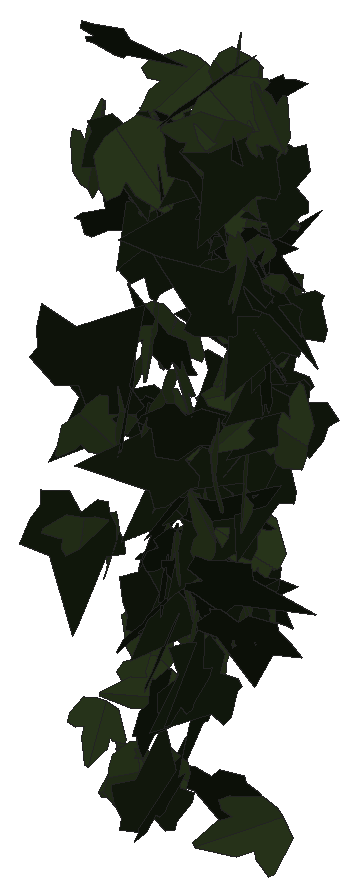
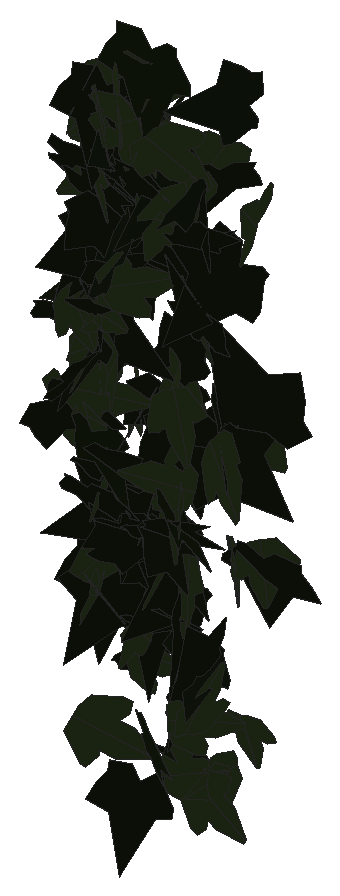
# SketchUp Ruby script. Lengths in inches.
U = 1.inch
M = Sketchup.active_model
def pt(a) = Geom::Point3d.new(a.map { |v| v * U })
def face(e, loops, mat)
  f = e.add_face(loops[0].map { |a| pt(a) })
  loops[1..].each { |l| e.add_face(l.map { |a| pt(a) }).erase! }
  f.material = f.back_material = mat if mat
  f
end
# faces: each face lists its corners as indices into pts; further lists are holes
def faces(e, pts, list, mat = nil) = list.each { |f| face(e, (f[0].is_a?(Array) ? f : [f]).map { |l| l.map { |i| pts[i] } }, mat) }
# xy, xz, yz: faces in a plane at the given z, y or x. An outline is a flat list of corners, or four numbers for a rectangle; further outlines are holes
def ring(l) = l.size == 4 ? [[l[0], l[1]], [l[2], l[1]], [l[2], l[3]], [l[0], l[3]]] : l.each_slice(2).to_a
def flat(e, list, mat, &to3) = list.each { |f| face(e, (f[0].is_a?(Array) ? f : [f]).map { |l| ring(l).map { |u, v| to3.(u, v) } }, mat) }
def xy(e, z, list, mat = nil) = flat(e, list, mat) { |x, y| [x, y, z] }
def xz(e, y, list, mat = nil) = flat(e, list, mat) { |x, z| [x, y, z] }
def yz(e, x, list, mat = nil) = flat(e, list, mat) { |y, z| [x, y, z] }
def lines(e, pts, list) = list.each { |a, b| e.add_line(pt(pts[a]), pt(pts[b])) }
# prism: a flat outline (further loops are holes) pulled along v
def prism(e, loops, v, mat = nil)
  f = face(e, loops, mat); d = Geom::Vector3d.new(v.map { |x| x * U })
  f.pushpull(f.normal.samedirection?(d) ? d.length : -d.length)
end
def box(e, o, s, mat = nil) = prism(e, [[o, [o[0] + s[0], o[1], o[2]], [o[0] + s[0], o[1] + s[1], o[2]], [o[0], o[1] + s[1], o[2]]]], [0, 0, s[2]], mat)
def at(x, y, z, deg = 0) = Geom::Transformation.translation(pt([x, y, z])) * Geom::Transformation.rotation(ORIGIN, Z_AXIS, deg.degrees)
def axes(o, x, y, z) = Geom::Transformation.new([*x, 0, *y, 0, *z, 0, *pt(o).to_a, 1])
def part(name) = M.definitions.add(name)
# library, detail: a bought-in or finely detailed component or shape, given as its bounding box
def library(name, o, s) = part(name).tap { |d| box(d.entities, o, s) }
def detail(e, o, s) = box(e.add_group.entities, o, s)
def put(e, d, t, mat = nil) = e.add_instance(d, t).tap { |i| i.material = mat if mat }
def group(e, t, mat = nil) = e.add_group.tap { |g| g.transformation = t; g.material = mat if mat }.entities
root = M.entities
M.materials.add("efeu1").color = [18, 25, 13]
M.materials.add("efeu2").color = [43, 57, 29]
c1 = part("ivyleaf_10")
p = [[0,0.5,-0.03],[-0.0625,2.02,-0.43],[-0.19,2.01,-0.46],[-0.54,1.05,-0.29],[-0.52,0.625,-0.18],[-0.83,0.76,-0.28],
  [-1.16,0.64,-0.33],[-1.15,0.33,-0.24],[-0.77,-0.39,0.02],[-0.3,-0.51,0.16],[0.04,-0.48,0.23],[-0.02,2.01,-0.4375],
  [-0.06,2.01,-0.43],[0.04,-0.49,0.23],[0.67,-0.49,0.14],[1.38,0.36,-0.2],[1.375,0.51,-0.24],[0.81,0.65,-0.19],
  [0.62,0.59,-0.15],[0.6,1.09,-0.28],[0.5,1.23,-0.31]]
faces(c1.entities,p,[[0,1,2,3,4,5,6,7,8,9,10],[11,12,0,13,14,15,16,17,18,19,20]],"efeu2")
c2 = part("ivyleaf_9")
p = [[1.54,2.16,1.25],[1.36,2.04,1.19],[-0.21,0.99,0.68],[-0.71,1.11,0.82],[-0.85,0.86,0.67],[-0.8,0.17,0.21],
  [-0.9,-0.01,0.1],[-0.67,-0.16,-0.02],[-0.08,-0.08,-0.05],[-0.03,-0.6,-0.4],[0.65,-0.88,-0.66],[0.83,-0.6,-0.49],
  [1.29,-0.42,-0.43],[1.8125,-0.07,-0.26],[1.21,0.44,0.15]]
faces(c2.entities,p,[[0,1,2,3,4,5,6,7,8,9,10,11,12,13,14]],"efeu1")
put(root,c1,axes([594.23,131.35,191.74],[-0.53643,-0.49083,0.10835],[-0.07654,-0.07685,-0.72708],[0.49678,-0.54184,0.00497]))
put(root,c1,axes([598.49,131.5,204.68],[-0.66643,-0.64585,0.35343],[-0.2321,-0.2681,-0.92759],[0.69868,-0.7051,0.02897]))
put(root,c1,axes([594.68,131.44,186.38],[0.71007,0,-0.05096],[-0.05096,0.00258,-0.71006],[0.00018,0.71189,0.00257]))
put(root,c2,axes([597.48,131.6,203.93],[0.44873,-0.83246,-0.02957],[-0.00604,0.03033,-0.94565],[0.83296,0.44868,0.00907]))
put(root,c1,axes([598.96,130.85,195.0625],[-0.07167,0.0519,1.0062],[-0.83234,0.56538,-0.08845],[-0.56775,-0.83541,0.00266]))
put(root,c2,axes([593.86,131.64,191.76],[-0.71749,-0.43155,-0.60235],[0.51539,0.31176,-0.83727],[0.53238,-0.88341,-0.00123]))
put(root,c1,axes([594.54,131.1,195.08],[-0.37758,-0.60266,-0.50523],[0.29373,0.41181,-0.71075],[0.7295,-0.47774,0.02468]))
put(root,c2,axes([597.78,130.88,188.04],[-0.66604,0.50161,-0.25033],[-0.19861,0.15239,0.8338],[0.52424,0.69502,-0.00215]))
put(root,c2,axes([599.1,131.86,204.14],[-0.72008,-0.57871,-0.0922],[0.06296,0.06882,-0.9237],[0.58262,-0.72269,-0.01414]))
put(root,c2,axes([593.99,131.54,195.82],[-0.4872,0.00001,1.14439],[0.98038,-0.64159,0.41738],[0.59032,1.06553,0.2513]))
put(root,c2,axes([597,130.87,184.61],[-0.54354,0.49023,-0.39924],[-0.2894,0.27518,0.7319],[0.56211,0.61571,-0.00923]))
put(root,c1,axes([595.88,131.08,203.49],[0.48219,0.75936,0.55764],[0.30038,0.46983,-0.89952],[-0.89295,0.5681,-0.00147]))
put(root,c1,axes([596.06,131.77,198.29],[0.57093,-0.39318,0.36943],[0.30649,-0.20628,-0.69321],[0.44399,0.64799,0.00348]))
put(root,c2,axes([597.36,132.16,201.05],[-0.18148,-0.23236,0.82745],[-0.56976,-0.60063,-0.29362],[0.64346,-0.59737,-0.02662]))
put(root,c2,axes([596.89,131.97,194.37],[-0.54453,-0.15865,0.72889],[-0.69816,-0.20942,-0.56716],[0.26271,-0.8854,0.00354]))
put(root,c2,axes([596.57,131.28,184.21],[-0.76186,0.12442,0.2214],[0.21886,-0.03354,0.77195],[0.12885,0.79267,-0.00208]))
put(root,c1,axes([599.74,131.8,184.8],[0.41186,0.20026,-0.86069],[-0.85151,-0.16391,-0.44561],[-0.23624,0.93997,0.10566]))
put(root,c2,axes([598.38,131.22,191.66],[0.80723,0.10253,0.55951],[0.55285,0.08718,-0.8136],[-0.13387,0.9783,0.01387]))
put(root,c2,axes([597.34,131.6,195.9],[0.27797,0.51142,-0.5665],[-0.27273,-0.49653,-0.58208],[-0.71281,0.38942,0.0018]))
put(root,c2,axes([598.68,131.9,199.3],[0.08396,0.03969,0.87475],[-0.87452,-0.04078,0.08579],[0.04443,-0.87782,0.03557]))
put(root,c1,axes([595.06,131.54,191.66],[0.34012,-0.55216,-0.36323],[-0.16634,0.32383,-0.64804],[0.63964,0.37782,0.02461]))
put(root,c2,axes([595.24,131.85,203.4375],[-0.17555,-0.661,-0.42038],[0.18438,0.38383,-0.68054],[0.76134,-0.24537,0.06788]))
put(root,c2,axes([598.67,132.15,204.16],[-0.87907,-0.24823,0.16724],[-0.16634,-0.02618,-0.91323],[0.24883,-0.89445,-0.01968]))
put(root,c2,axes([597.71,132.43,188.16],[-0.40711,-0.56027,0.44435],[-0.27357,-0.35039,-0.69244],[0.66069,-0.49032,-0.01292]))
put(root,c2,axes([598.15,131.2,205.79],[0.05078,1.00163,0.2455],[-0.14956,0.25035,-0.99049],[-1.02038,0.01316,0.1574]))
put(root,c1,axes([598.92,131.79,200.91],[0.56049,-0.62433,-0.35969],[-0.22076,0.28498,-0.83867],[0.68588,0.60192,0.02399]))
put(root,c1,axes([598.3125,131.94,204.35],[0.88329,0.30052,-0.02109],[-0.01838,-0.01147,-0.933],[-0.3007,0.88347,-0.00494]))
put(root,c2,axes([596.37,131.375,187.28],[0.06423,-0.06962,-0.79537],[-0.56148,0.56336,-0.09465],[0.56763,0.56513,-0.00363]))
put(root,c2,axes([596.53,131.99,197.18],[0.39757,-0.33743,0.58633],[-0.45285,0.37249,0.52142],[-0.50257,-0.60257,-0.006]))
put(root,c2,axes([595.58,131.43,195.68],[-0.17426,0.0591,-0.95216],[-0.8977,0.31742,0.18399],[0.32286,0.91445,-0.00233]))
put(root,c1,axes([595.26,131.58,195.36],[0.22783,-0.39312,-0.61424],[-0.04583,0.63453,-0.4231],[0.72783,0.16301,0.16563]))
put(root,c2,axes([596.55,131.4,188.48],[-0.03502,0.43001,0.66659],[-0.02145,0.66648,-0.43107],[-0.79296,-0.03702,-0.01778]))
put(root,c1,axes([595.18,131.55,184.77],[-0.06549,-0.15586,-0.70183],[0.30076,0.63417,-0.1689],[0.653,-0.30772,0.0074]))
put(root,c1,axes([596.43,131.79,196.15],[0.05812,-0.64739,-0.44053],[-0.0012,0.44166,-0.64922],[0.78305,0.04872,0.0317]))
put(root,c2,axes([594.33,131.88,205.82],[0.64296,-0.14555,0.45431],[0.47036,0.06607,-0.6445],[0.07968,0.7845,0.13857]))
put(root,c1,axes([597.14,132.51,204.38],[0.40863,-0.76731,0.42353],[0.21062,-0.36764,-0.86926],[0.85076,0.45956,0.01177]))
put(root,c1,axes([594.24,131.5,202.07],[-0.05751,0.57676,-0.73354],[-0.08736,0.72837,0.57955],[0.92903,0.1042,0.00909]))
put(root,c1,axes([598.35,131.72,205.39],[0.3547,0.64192,0.56881],[0.25545,0.50853,-0.73318],[-0.81875,0.43675,0.01767]))
put(root,c2,axes([594.67,132.56,195.28],[0.06409,0.31215,-0.93065],[-0.24641,-0.89765,-0.31806],[-0.95018,0.25385,0.0197]))
put(root,c2,axes([596.09,131.86,202.91],[0.15249,0.05484,-0.92547],[-0.92423,0.08265,-0.14738],[0.07281,0.9343,0.06736]))
put(root,c2,axes([598.85,131.94,190.23],[0.68222,0.51339,-0.45747],[-0.3829,-0.25165,-0.85342],[-0.57117,0.7819,0.0257]))
put(root,c1,axes([595.47,132.32,184.33],[-0.41713,-0.07572,0.75812],[-0.74073,-0.16199,-0.42374],[0.17832,-0.85,0.01322]))
put(root,c1,axes([598.69,132.22,204.17],[-0.85295,0.31445,0.19322],[-0.23063,-0.07428,-0.89723],[-0.28813,-0.8714,0.1462]))
put(root,c1,axes([596.54,132.28,196.9],[-0.63065,0.60577,-0.2107],[0.14205,-0.15624,-0.87435],[-0.62544,-0.6463,0.01388]))
put(root,c1,axes([596.25,132.4375,184.72],[-0.19713,-0.02686,-0.75741],[-0.75665,-0.03768,0.19826],[-0.04325,0.78174,-0.01647]))
put(root,c2,axes([599.07,132.88,199.07],[-0.52671,-0.71516,0.08034],[0.02712,-0.11922,-0.88339],[0.71914,-0.5193,0.09216]))
put(root,c1,axes([597.79,131.86,203.08],[-0.3478,0.50117,0.6409],[-0.44282,0.46811,-0.60636],[-0.68252,-0.5591,0.06681]))
put(root,c2,axes([596.29,132.19,195.38],[0.35336,0.53975,-0.61882],[-0.56617,-0.32779,-0.60921],[-0.59474,0.63274,0.21227]))
put(root,c2,axes([598.24,133.0625,203.69],[-0.06951,-0.29116,0.81802],[0.08504,-0.81898,-0.28428],[0.86412,0.05717,0.09377]))
put(root,c1,axes([595.73,132.82,186.66],[0.03721,0.01773,0.81143],[-0.56244,-0.58506,0.03858],[0.58515,-0.56348,-0.01452]))
put(root,c1,axes([597.23,132.67,191.95],[-0.44315,0.71475,0.31559],[0.15909,-0.27267,0.84094],[0.76495,0.47078,0.00793]))
put(root,c1,axes([598.35,132.63,200.94],[-0.90983,-0.09972,0.23756],[0.23602,0.02702,0.91528],[-0.10331,0.93994,-0.00111]))
put(root,c2,axes([595.76,133.09,201.8],[-0.76704,-0.5943,-0.02832],[0.02062,0.01963,-0.97033],[0.59461,-0.76731,-0.00289]))
put(root,c2,axes([594.55,132.01,200.82],[0.69212,0.68083,0.29912],[0.19239,0.23078,-0.97044],[-0.71832,0.71781,0.02829]))
put(root,c1,axes([598.26,132.35,202.57],[0.31984,0.211,0.87574],[0.70789,0.51584,-0.38282],[-0.55708,0.77662,0.01634]))
put(root,c1,axes([598.5625,133.2,195.89],[0.19326,0.3552,-0.76719],[-0.38379,-0.66435,-0.40427],[-0.75329,0.4296,0.00915]))
put(root,c1,axes([599.28,132.79,204.23],[-0.20636,0.83209,0.16717],[0.03273,-0.16412,0.85727],[0.84809,0.2088,0.0076]))
put(root,c2,axes([596.5,133.1875,200.86],[-0.46227,-0.51532,-0.47286],[-0.1225,-0.49839,0.6629],[-0.68858,0.43462,0.19952]))
put(root,c2,axes([596.97,132.48,190.39],[0.70793,0.21976,-0.8054],[-0.80265,-0.11126,-0.73587],[-0.22961,1.06651,0.08919]))
put(root,c1,axes([596.01,133.24,202.25],[0.22349,0.53159,-0.65896],[-0.33023,-0.57282,-0.5741],[-0.7796,0.39503,0.05428]))
put(root,c2,axes([599.71,132.96,202.83],[-0.80086,0.15449,0.41787],[-0.40877,0.08702,-0.81559],[-0.17716,-0.89912,-0.00714]))
put(root,c1,axes([594.31,133.09,195.44],[0.13296,-0.95533,0.15934],[0.00185,-0.16059,-0.96433],[0.96852,0.13146,-0.02004]))
put(root,c2,axes([595.17,132.71,198.88],[-0.56776,0.43593,0.54936],[0.39333,-0.38725,0.7138],[0.58062,0.68861,0.05364]))
put(root,c1,axes([596.3,132.85,191.2],[-0.28976,0.86865,-0.11984],[0.01712,-0.12058,-0.91544],[-0.87671,-0.28945,0.02173]))
put(root,c1,axes([595.63,132.9,203.13],[0.35766,0.91453,-0.09404],[-0.01874,-0.09364,-0.98184],[-0.91917,0.35776,-0.01657]))
put(root,c1,axes([598.43,133.28,198.14],[0.29211,0.58127,-0.60954],[-0.36853,-0.49192,-0.64572],[-0.75737,0.46355,0.07911]))
put(root,c2,axes([596.2,132.92,192.53],[-0.41821,0.7609,-0.37313],[0.15779,-0.3389,-0.86795],[-0.83265,-0.4464,0.02292]))
put(root,c1,axes([597.68,132.87,204.5],[-0.43554,-0.01015,-0.81873],[0.81688,-0.06876,-0.4337],[-0.05596,-0.92481,0.04123]))
put(root,c2,axes([598.65,133.0625,199.59],[0.56227,-0.69001,0.09687],[0.17142,0.01633,-0.87863],[0.67536,0.57032,0.14236]))
put(root,c1,axes([598.32,133.23,198.19],[0.34606,0.64987,-0.48786],[-0.22691,-0.43189,-0.73627],[-0.78029,0.41381,-0.00226]))
put(root,c2,axes([597.31,133.39,192.45],[-0.84135,-0.44479,-0.05657],[0.05854,0.01028,-0.95151],[0.44454,-0.84318,0.01824]))
put(root,c2,axes([595.36,132.375,188.875],[0.07212,0.76052,0.31916],[-0.00243,0.32058,-0.76333],[-0.82477,0.06556,0.03016]))
put(root,c2,axes([598.27,132.97,201.83],[0.10994,0.6776,-0.55936],[-0.14707,-0.54157,-0.68497],[-0.86625,0.17795,0.0453]))
put(root,c2,axes([595.76,132.7,203.45],[0.98827,-0.04104,-0.0708],[-0.06884,0.04707,-0.98814],[0.04425,0.98969,0.04406]))
put(root,c2,axes([599.07,132.63,196.71],[0.0939,-0.17142,0.87532],[-0.22855,0.84614,0.19023],[-0.86216,-0.24298,0.0449]))
put(root,c1,axes([597.19,133.03,188.3],[0.17854,0.05805,0.81988],[-0.81084,-0.12494,0.18542],[0.13459,-0.82974,0.02944]))
put(root,c2,axes([596.42,133.47,189.84],[-0.85406,-0.30228,0.06457],[-0.05066,-0.05028,-0.90547],[0.30492,-0.85502,0.03042]))
put(root,c2,axes([598.21,132.64,200.92],[0.82853,0.36897,0.02611],[0.02071,0.01767,-0.90694],[-0.36931,0.82875,0.00771]))
put(root,c2,axes([595.92,133.31,193.81],[-0.71016,0.39382,-0.48971],[0.41931,-0.25346,-0.8119],[-0.46807,-0.82457,0.01567]))
put(root,c2,axes([598.53,132.64,205.18],[0.253,0.90116,-0.0483],[-0.03397,-0.04062,-0.93575],[-0.90182,0.25434,0.0217]))
put(root,c2,axes([598.18,133.07,198.29],[-0.24013,0.10546,-0.90134],[-0.82585,-0.41188,0.17183],[-0.37617,0.83692,0.19814]))
put(root,c1,axes([597.92,133.52,193.78],[-0.14552,0.52565,-0.67132],[0.16319,-0.65126,-0.54532],[-0.83686,-0.2184,0.0104]))
put(root,c2,axes([597.4375,133.45,203.4375],[-0.92216,-0.12921,-0.2486],[0.2492,0.01254,-0.93092],[0.12804,-0.955,0.02141]))
put(root,c2,axes([598.62,133.41,202.72],[-0.90631,-0.08978,-0.12887],[0.12661,0.02895,-0.9106],[0.09294,-0.91497,-0.01617]))
put(root,c1,axes([596.11,133.38,204.64],[0.63454,0.32422,-0.62424],[-0.5764,-0.2422,-0.71171],[-0.40318,0.85654,0.03504]))
put(root,c1,axes([594.95,133.28,187.17],[-0.01853,0.82433,0.30778],[-0.00119,-0.30787,0.8245],[0.87991,0.01694,0.00759]))
put(root,c2,axes([598.25,132.45,203.64],[0.11625,0.35827,0.78626],[0.03938,0.79033,-0.36594],[-0.86314,0.08431,0.0892]))
put(root,c2,axes([597.42,133.57,200.49],[-0.67536,-0.65984,-0.16469],[0.09996,0.13328,-0.94386],[0.67269,-0.68226,-0.0251]))
put(root,c2,axes([598.5,133.14,203.98],[-0.26282,-0.0857,-0.87804],[-0.81926,-0.31617,0.27609],[-0.32728,0.86027,0.01399]))
put(root,c2,axes([596.09,133.78,193],[-0.8145,-0.43484,0.17482],[-0.05018,-0.2676,-0.8994],[0.46597,-0.7889,0.20872]))
put(root,c1,axes([598.11,133.71,190.18],[0.01918,0.4415,-0.73467],[-0.03565,-0.7338,-0.44191],[-0.85638,0.04044,0.00194]))
put(root,c1,axes([598.42,132.84,190.22],[-0.41874,0.55679,0.42577],[-0.26709,0.3318,-0.69657],[-0.64804,-0.49652,0.01197]))
put(root,c2,axes([597.05,133.1,192.14],[0.68881,0.54607,-0.17039],[0.1278,0.11305,0.87896],[0.55758,-0.70051,0.00902]))
put(root,c1,axes([598.38,133.56,196.36],[0.25952,0.09658,-0.82508],[-0.74993,-0.34459,-0.27621],[-0.35733,0.79332,-0.01953]))
put(root,c1,axes([595.5,133.02,191.49],[-0.74757,0.28675,0.34177],[-0.3236,0.11056,-0.8006],[-0.30711,-0.81452,0.01165]))
put(root,c2,axes([598.39,132.97,198.27],[0.85606,-0.15122,-0.43957],[-0.43116,0.08602,-0.86927],[0.17375,0.95846,0.00866]))
put(root,c1,axes([598.05,132.84,205.48],[-0.27034,0.34773,0.74608],[-0.6525,0.3882,-0.41736],[-0.5018,-0.69212,0.14075]))
put(root,c1,axes([598.35,133.18,205.06],[0.45487,-0.71845,-0.31869],[-0.17083,0.26903,-0.85034],[0.76717,0.48589,-0.00039]))
put(root,c2,axes([598.625,133.17,190.22],[-0.62354,0.46457,0.21404],[-0.18089,0.1154,-0.77743],[-0.47845,-0.64907,0.01498]))
put(root,c1,axes([598.78,133.06,198.74],[0.08189,-0.01313,-0.8836],[-0.76816,0.43763,-0.0777],[0.43686,0.77197,0.02902]))
put(root,c2,axes([598.79,134.02,196.68],[-0.35797,-0.57022,0.55203],[-0.23177,-0.50408,-0.67098],[0.75906,-0.42283,0.05546]))
put(root,c1,axes([596.54,133.75,189.6],[0.06424,0.55084,-0.5505],[-0.084,-0.54424,-0.55439],[-0.77422,0.10476,0.01447]))
put(root,c2,axes([595.58,132.83,190.94],[0.52013,0.51175,0.34844],[0.25282,0.23985,-0.72965],[-0.56514,0.57829,-0.00572]))
put(root,c1,axes([597.24,133.75,199.98],[0.14296,0.23367,0.83932],[-0.60075,-0.58956,0.26646],[0.63099,-0.61425,0.06353]))
put(root,c2,axes([597.9375,133.83,194.45],[-0.87525,-0.15672,0.29435],[-0.27963,-0.10553,-0.88766],[0.18169,-0.91737,0.05183]))
put(root,c1,axes([599.62,133.3,195.36],[0.15059,0.16574,0.93824],[-0.95239,-0.00062,0.15297],[0.02689,-0.95025,0.16355]))
put(root,c2,axes([598.36,133.24,195.01],[-0.40158,0.76426,-0.05938],[0.00992,-0.06185,-0.86311],[-0.7665,-0.4012,0.01994]))
put(root,c2,axes([597.26,133.9375,200.73],[0.29389,-0.53712,0.65414],[0.29578,-0.58363,-0.6121],[0.79305,0.41672,-0.01412]))
put(root,c2,axes([598.96,133.9375,198.9],[-0.66242,-0.5785,-0.1295],[0.17323,-0.00317,-0.8719],[0.56695,-0.67495,0.11509]))
put(root,c1,axes([597.18,133.57,205.05],[-0.49476,0.10545,-0.74982],[0.70359,-0.26703,-0.5018],[-0.27986,-0.85774,0.06404]))
put(root,c2,axes([596.78,134.18,195.45],[0.44028,-0.50963,-0.6154],[0.41677,-0.45301,0.67333],[-0.68172,-0.60609,0.01419]))
put(root,c1,axes([598.41,133.5,203.47],[0.65044,-0.55992,-0.23318],[-0.1706,0.15921,-0.85819],[0.58204,0.67238,0.00903]))
put(root,c2,axes([596.26,133.8,186.52],[-0.52836,0.10109,-0.57915],[0.54388,-0.21159,-0.53312],[-0.22321,-0.75486,0.07187]))
put(root,c2,axes([599.29,134.02,195.875],[-0.03861,-0.00353,-0.81943],[-0.02577,-0.81993,0.00475],[-0.81904,0.02597,0.03848]))
put(root,c1,axes([598.13,133.78,191],[0.05088,0.61239,0.52206],[-0.21517,-0.4937,0.60009],[0.77541,-0.17717,0.13227]))
put(root,c2,axes([598.8125,132.8,200.34],[-0.23923,0.57821,-0.62484],[-0.3024,0.54899,0.62381],[0.7958,0.38243,0.04921]))
put(root,c1,axes([595.7,133.23,193.8],[-0.58455,0.37335,0.53244],[-0.47349,0.24638,-0.6926],[-0.44575,-0.75133,0.03746]))
put(root,c2,axes([596.92,133.26,184.49],[0.63947,0.44654,-0.35475],[-0.29361,-0.19914,-0.77994],[-0.48891,0.70364,0.00439]))
put(root,c1,axes([597.42,133.81,197.68],[-0.51521,0.4824,-0.55928],[0.28854,-0.49625,-0.69384],[-0.67988,-0.57616,0.12935]))
put(root,c1,axes([598.66,133.84,199.1875],[-0.15999,-0.77396,0.24193],[-0.03497,-0.23978,-0.7902],[0.81013,-0.1632,0.01367]))
put(root,c1,axes([595.46,133.31,194.25],[-0.13317,-0.10252,0.8129],[0.6375,0.50439,0.16805],[-0.5147,0.65126,-0.00218]))
put(root,c2,axes([594.9,133.29,188.63],[-0.2352,-0.4745,0.78731],[0.32939,0.71521,0.52944],[-0.8582,0.40454,-0.01257]))
put(root,c2,axes([595.47,133.21,190.22],[0.07403,-0.04347,-0.87338],[-0.76661,0.41847,-0.08581],[0.42071,0.77017,-0.00268]))
put(root,c1,axes([595.39,133.64,196.96],[-0.75047,-0.03693,0.36902],[-0.3672,-0.04282,-0.75105],[0.05201,-0.83519,0.02219]))
put(root,c2,axes([597.99,134.05,193.61],[-0.69426,-0.34169,-0.37691],[0.38728,0.05853,-0.76642],[0.32989,-0.78781,0.10653]))
put(root,c2,axes([597.68,133.24,190.36],[0.68556,0.54044,0.04093],[0.03022,0.02777,-0.87296],[-0.54115,0.68622,0.0031]))
